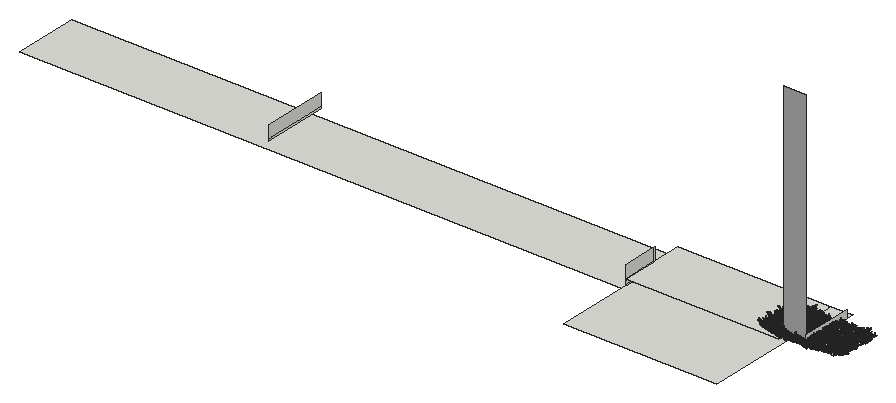
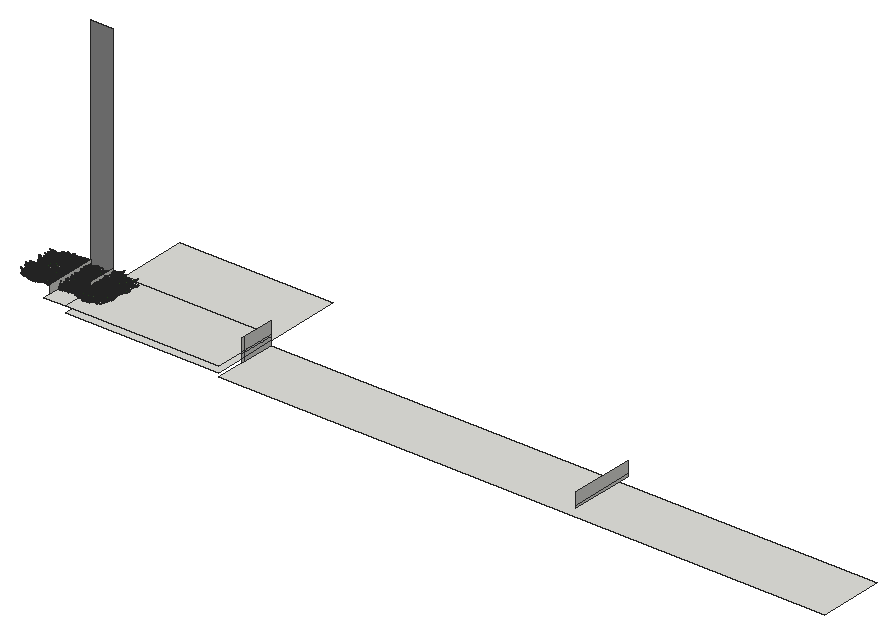
# SketchUp Ruby script. Lengths in inches.
U = 1.inch
M = Sketchup.active_model
def pt(a) = Geom::Point3d.new(a.map { |v| v * U })
def face(e, loops, mat)
  f = e.add_face(loops[0].map { |a| pt(a) })
  loops[1..].each { |l| e.add_face(l.map { |a| pt(a) }).erase! }
  f.material = f.back_material = mat if mat
  f
end
# faces: each face lists its corners as indices into pts; further lists are holes
def faces(e, pts, list, mat = nil) = list.each { |f| face(e, (f[0].is_a?(Array) ? f : [f]).map { |l| l.map { |i| pts[i] } }, mat) }
# xy, xz, yz: faces in a plane at the given z, y or x. An outline is a flat list of corners, or four numbers for a rectangle; further outlines are holes
def ring(l) = l.size == 4 ? [[l[0], l[1]], [l[2], l[1]], [l[2], l[3]], [l[0], l[3]]] : l.each_slice(2).to_a
def flat(e, list, mat, &to3) = list.each { |f| face(e, (f[0].is_a?(Array) ? f : [f]).map { |l| ring(l).map { |u, v| to3.(u, v) } }, mat) }
def xy(e, z, list, mat = nil) = flat(e, list, mat) { |x, y| [x, y, z] }
def xz(e, y, list, mat = nil) = flat(e, list, mat) { |x, z| [x, y, z] }
def yz(e, x, list, mat = nil) = flat(e, list, mat) { |y, z| [x, y, z] }
def lines(e, pts, list) = list.each { |a, b| e.add_line(pt(pts[a]), pt(pts[b])) }
# prism: a flat outline (further loops are holes) pulled along v
def prism(e, loops, v, mat = nil)
  f = face(e, loops, mat); d = Geom::Vector3d.new(v.map { |x| x * U })
  f.pushpull(f.normal.samedirection?(d) ? d.length : -d.length)
end
def box(e, o, s, mat = nil) = prism(e, [[o, [o[0] + s[0], o[1], o[2]], [o[0] + s[0], o[1] + s[1], o[2]], [o[0], o[1] + s[1], o[2]]]], [0, 0, s[2]], mat)
def at(x, y, z, deg = 0) = Geom::Transformation.translation(pt([x, y, z])) * Geom::Transformation.rotation(ORIGIN, Z_AXIS, deg.degrees)
def axes(o, x, y, z) = Geom::Transformation.new([*x, 0, *y, 0, *z, 0, *pt(o).to_a, 1])
def part(name) = M.definitions.add(name)
# library, detail: a bought-in or finely detailed component or shape, given as its bounding box
def library(name, o, s) = part(name).tap { |d| box(d.entities, o, s) }
def detail(e, o, s) = box(e.add_group.entities, o, s)
def put(e, d, t, mat = nil) = e.add_instance(d, t).tap { |i| i.material = mat if mat }
def group(e, t, mat = nil) = e.add_group.tap { |g| g.transformation = t; g.material = mat if mat }.entities
root = M.entities
M.materials.add("Material82").color = [68, 110, 58]
M.materials.add("Material83").color = [48, 90, 38]
M.materials.add("Material84").color = [68, 110, 48]
M.materials.add("Material85").color = [48, 90, 48]
M.materials.add("Material86").color = [58, 110, 58]
M.materials.add("Material87").color = [58, 90, 38]
M.materials.add("Material88").color = [68, 100, 58]
M.materials.add("Material89").color = [48, 100, 38]
M.materials.add("[Color M03]1").color = [170, 170, 170]
c1 = part("grass00")
p = [[-0.6875,0.15,0],[-0.56,0.08,5.52],[-0.04,0.03,2.76],[0.48,-0.02,0],[0.35,-0.02,5.52],[-0.1,-0.14,5.52],
  [-0.12,0.65,8.37],[-0.42,0.65,8.37]]
faces(c1.entities,p,[[0,1,2,3],[3,2,4],[1,5,2],[5,4,2],[1,6,5],[4,5,6],[7,6,1]])
c2 = part("Group16\#1")
put(c2.entities,c1,axes([1.44,-0.61,-0.01],[0.05352,0.12609,0],[-0.10704,0.04543,0.07239],[0.06664,-0.02828,0.11628]),"Material85")
put(c2.entities,c1,axes([0.76,-0.15,-0.01],[0.04676,0.24062,0],[-0.23162,0.04501,0.06642],[0.0652,-0.01267,0.23595]),"Material82")
put(c2.entities,c1,axes([0.79,0.01,-0.01],[-0.00606,0.34651,0],[-0.34381,-0.00602,0.0432],[0.04319,0.00076,0.34386]))
put(c2.entities,c1,axes([1,0.23,-0.01],[-0.07192,0.31144,0],[-0.28722,-0.06632,0.1236],[0.12043,0.02781,0.29478]),"Material84")
put(c2.entities,c1,axes([1.66,0.77,-0.01],[-0.13828,0.29651,0],[-0.21551,-0.1005,0.22471],[0.20365,0.09498,0.23779]),"Material89")
put(c2.entities,c1,axes([0.6875,0.52,-0.01],[-0.18126,0.24051,0],[-0.22746,-0.17142,0.09788],[0.07817,0.05891,0.28481]),"Material84")
put(c2.entities,c1,axes([0.68,0.78,-0.01],[-0.215,0.18688,0],[-0.12385,-0.14248,0.21334],[0.13995,0.16101,0.18878]),"Material82")
put(c2.entities,c1,axes([0.56,1,-0.01],[-0.13756,0.07624,0],[-0.06159,-0.11112,0.0927],[0.04494,0.08108,0.12705]),"Material84")
put(c2.entities,c1,axes([0.2,0.64,-0.01],[-0.23729,0.07254,0],[-0.05711,-0.18681,0.153],[0.04473,0.14632,0.19535]),"Material89")
put(c2.entities,c1,axes([0.0625,0.72,-0.01],[-0.28874,0.02525,0],[-0.02179,-0.24916,0.14647],[0.01276,0.14591,0.25012]),"Material82")
put(c2.entities,c1,axes([-0.08,0.62,-0.01],[-0.34089,-0.04187,0],[0.03255,-0.26504,0.216],[-0.02633,0.21439,0.26703]),"Material89")
put(c2.entities,c1,axes([-0.34,0.98,-0.01],[-0.14314,-0.0493,0],[0.04397,-0.12769,0.06843],[-0.02228,0.0647,0.13505]),"Material89")
put(c2.entities,c1,axes([-0.87,1.45,-0.01],[-0.23488,-0.14114,0],[0.13761,-0.22901,0.06087],[-0.03135,0.05217,0.26717]))
put(c2.entities,c1,axes([-0.72,0.77,-0.01],[-0.14208,-0.13251,0],[0.07209,-0.0773,0.16301],[-0.11118,0.11922,0.1057]),"Material89")
put(c2.entities,c1,axes([-0.62,0.43,-0.01],[-0.14845,-0.21203,0],[0.18654,-0.13061,0.12304],[-0.10079,0.07057,0.22772]),"Material82")
put(c2.entities,c1,axes([-0.68,0.29,-0.01],[-0.13639,-0.32136,0],[0.31723,-0.13464,0.05579],[-0.05136,0.0218,0.34462]),"Material83")
put(c2.entities,c1,axes([-0.64,0.125,-0.01],[-0.0458,-0.23569,0],[0.22124,-0.043,0.08276],[-0.08124,0.01579,0.22538]),"Material86")
put(c2.entities,c1,axes([-1.6,-0.03,-0.01],[0.00576,-0.32897,0],[0.27526,0.00482,0.18018],[-0.18015,-0.00315,0.2753]),"Material84")
put(c2.entities,c1,axes([-1.36,-0.31,-0.01],[0.05718,-0.24765,0],[0.18172,0.04196,0.17267],[-0.16825,-0.03885,0.1865]),"Material89")
put(c2.entities,c1,axes([-1.54,-0.72,-0.01],[0.06537,-0.14017,0],[0.13555,0.06321,0.03939],[-0.0357,-0.01665,0.14956]))
put(c2.entities,c1,axes([-1.19,-0.9,-0.01],[0.09597,-0.12735,0],[0.11214,0.08451,0.07557],[-0.06035,-0.04548,0.14042]),"Material88")
put(c2.entities,c1,axes([-0.47,-0.54,-0.01],[0.11588,-0.10072,0],[0.0618,0.0711,0.12124],[-0.07953,-0.0915,0.0942]))
put(c2.entities,c1,axes([-0.47,-0.84,-0.01],[0.11927,-0.0661,0],[0.06603,0.11913,0.00646],[-0.00313,-0.00565,0.13621]),"Material84")
put(c2.entities,c1,axes([-0.38,-1.24,-0.01],[0.28037,-0.08571,0],[0.0618,0.20215,0.20315],[-0.05939,-0.19428,0.21139]),"Material88")
put(c2.entities,c1,axes([-0.06,-0.66,-0.01],[0.22719,-0.01987,0],[0.01247,0.14255,0.17758],[-0.01547,-0.17691,0.1431]),"Material87")
put(c2.entities,c1,axes([0.11,-0.89,-0.01],[0.14882,0.01828,0],[-0.01058,0.08611,0.12229],[0.01491,-0.12138,0.08676]),"Material85")
put(c2.entities,c1,axes([0.25,-0.72,-0.01],[0.20481,0.07053,0],[-0.06206,0.18022,0.10291],[0.03351,-0.0973,0.1906]),"Material85")
put(c2.entities,c1,axes([0.85,-1.42,-0.01],[0.16481,0.09904,0],[-0.09472,0.15762,0.05616],[0.02893,-0.04814,0.18389]),"Material84")
put(c2.entities,c1,axes([1.01,-1.09,-0.01],[0.21858,0.20385,0],[-0.17495,0.1876,0.15339],[0.10462,-0.11218,0.25652]),"Material89")
put(c2.entities,c1,axes([1.01,-0.71,-0.01],[0.08733,0.12473,0],[-0.06445,0.04512,0.13037],[0.1068,-0.07477,0.07867]),"Material85")
c3 = part("Group15\#1")
put(c3.entities,c2,at(0,0,0))
c4 = part("3darcstudiotree_grass00\#1")
put(c4.entities,c3,at(0,0,0))
xy(root,-42.1875,[[1048.66,335.84,1534.73,387.84]])
xy(root,-39.125,[[1534.73,273.41,1657.41,387.84]])
xy(root,-34.17,[[1534.73,335.84,1657.41,387.84],[1657.41,341.03,1674.99,387.84]])
xz(root,341.03,[[1657.41,-34.17,1674.99,144.9375]],"[Color M03]1")
yz(root,1248.34,[[335.84,-35.625,387.84,-34.17],[335.84,-34.17,387.84,-24.25]])
yz(root,1534.73,[[335.84,-42.1875,362.97,-39.125],[362.97,-42.1875,364.46,-39.125],[335.84,-39.125,362.97,-35.625],[362.97,-39.125,364.46,-35.625],[335.84,-35.625,362.97,-34.17],
  [362.97,-35.625,364.46,-34.17],[335.84,-34.17,362.97,-24.25],[362.97,-34.17,364.46,-24.25]])
yz(root,1657.41,[[341.03,-34.17,362.97,-27.66]])
yz(root,1674.99,[[341.03,-34.17,381.72,-27.66]])
put(root,c4,axes([1645.09,350.95,-34.17],[-3.06097,-0.5879,0],[1.66705,-1.34995,-0.03924],[0.1162,-0.0941,1.93013]))
put(root,c4,axes([1646.65,355.5625,-34.17],[-4.03652,-0.16228,0],[0.44348,-1.71564,-0.03002],[0.01485,-0.05745,1.59842]))
put(root,c4,axes([1646.35,360.35,-34.17],[2.89762,-1.1399,0],[2.43274,0.96179,-0.0036],[0.01556,0.00615,1.5794]))
put(root,c4,axes([1646.26,342.71,-34.17],[3.9501,-0.3019,0],[0.82816,1.68526,-0.01483],[0.01308,0.02661,1.51152]))
put(root,c4,axes([1645.96,364.46,-34.17],[3.35543,0.83331,0],[-2.02345,1.2672,-0.03908],[-0.13338,0.08353,1.82303]))
put(root,c4,axes([1646.7,348.62,-34.17],[2.855,1.42821,0],[-2.79418,0.86872,-0.04305],[-0.19263,0.05989,1.51958]))
put(root,c4,axes([1648.4,371.03,-34.17],[4.14496,0.31804,0],[-0.83759,1.6978,-0.03864],[-0.04159,0.0843,1.85268]))
put(root,c4,axes([1648.57,342.22,-34.17],[3.14768,1.20624,0],[-3.13864,1.27383,-0.06236],[-0.23969,0.09728,1.86199]))
put(root,c4,axes([1649.89,367.78,-34.17],[1.22629,-1.22817,0],[3.78204,0.58732,-0.0431],[0.18193,0.02825,1.38217]))
put(root,c4,axes([1649.94,354.84,-34.17],[2.09831,-1.02697,0],[3.53268,1.1226,-0.04335],[0.15343,0.04876,1.54559]))
put(root,c4,axes([1649.82,351.3,-34.17],[-2.72452,1.24598,0],[-3.55259,-1.2082,-0.04683],[-0.18808,-0.06396,1.86493]))
put(root,c4,axes([1649.3,357.3125,-34.17],[3.77194,0.53127,0],[-1.56854,1.73204,-0.02984],[-0.04464,0.0493,1.55474]))
put(root,c4,axes([1650.93,353.18,-34.17],[0.71144,-1.32945,0],[4.31841,0.35942,-0.04294],[0.17046,0.01419,1.34209]))
put(root,c4,axes([1651.22,360.26,-34.17],[1.7149,-1.22637,0],[3.67075,0.79833,-0.00061],[0.00329,0.00072,1.94394]))
put(root,c4,axes([1651.55,362.27,-34.17],[1.13517,-1.33714,0],[4.08386,0.53922,-0.04023],[0.16123,0.02129,1.36415]))
put(root,c4,axes([1650.625,366.27,-34.17],[-1.96155,1.42232,0],[-3.86474,-0.82896,-0.01158],[-0.04562,-0.00979,1.47884]))
put(root,c4,axes([1652.02,372.46,-34.17],[-0.47401,-1.83018,0],[3.81106,-0.15352,-0.01024],[0.06486,-0.00261,1.82793]))
put(root,c4,axes([1651.45,363.91,-34.17],[-2.22727,1.60419,0],[-4.12877,-0.89155,-0.00813],[-0.02667,-0.00576,1.31962]))
put(root,c4,axes([1651.8,348.36,-34.17],[-2.60888,1.40075,0],[-3.4553,-1.0009,-0.02364],[-0.11495,-0.0333,1.93862]))
put(root,c4,axes([1652.17,347.26,-34.17],[3.43972,-1.19732,0],[3.07284,1.37298,-0.00351],[0.01073,0.00479,1.60808]))
put(root,c4,axes([1652.2,344.94,-34.17],[2.57433,-1.10368,0],[3.03991,1.10279,-0.05921],[0.27011,0.09799,1.91907]))
put(root,c4,axes([1654.11,364.41,-34.17],[-1.00872,-1.50256,0],[3.76018,-0.39261,-0.00114],[0.00668,-0.0007,1.77079]))
put(root,c4,axes([1654.41,351.03,-34.17],[-4.39065,-0.68044,0],[1.48247,-1.48779,-0.03326],[0.06181,-0.06203,1.54402]))
put(root,c4,axes([1654.4,365.79,-34.17],[-4.44259,0.07323,0],[-0.15396,-1.45277,-0.02048],[-0.00618,-0.05831,1.99696]))
put(root,c4,axes([1653.9,361.58,-34.17],[-2.76199,0.84111,0],[-2.40625,-1.22891,-0.02049],[-0.06035,-0.03082,1.42185]))
put(root,c4,axes([1654.5,344.48,-34.17],[4.22079,-0.16227,0],[0.44484,1.79962,-0.00515],[0.00263,0.01065,1.80879]))
put(root,c4,axes([1656.62,341.46,-34.17],[-4.16244,-0.15093,0],[0.36502,-1.56574,-0.01686],[0.00714,-0.03063,1.38194]))
put(root,c4,axes([1655.3,358.125,-34.17],[-0.6643,1.32662,0],[-4.47997,-0.3489,-0.01512],[-0.08059,-0.00628,1.85999]))
put(root,c4,axes([1656.86,349.27,-34.17],[0.943,-1.41783,0],[3.80413,0.39351,-0.01105],[0.05525,0.00572,1.52421]))
put(root,c4,axes([1655.42,340.13,-34.17],[0.93193,1.68006,0],[-3.63506,0.3136,-0.00261],[-0.01526,0.00132,1.6704]))
put(root,c4,axes([1657.5,355.56,-34.17],[-3.93808,-0.75827,0],[2.05575,-1.66052,-0.06565],[0.13947,-0.11266,1.70067]))
put(root,c4,axes([1655.9,359.26,-34.17],[-0.07538,1.68656,0],[-4.43832,-0.03085,-0.00958],[-0.0427,-0.0003,1.48335]))
put(root,c4,axes([1656.73,347.11,-34.17],[0.31598,1.50106,0],[-3.48689,0.11416,-0.00998],[-0.05116,0.00168,1.34846]))
put(root,c4,axes([1657.55,371.18,-34.17],[3.02082,-1.15648,0],[2.42176,0.98385,-0.02978],[0.11407,0.04634,1.43312]))
put(root,c4,axes([1657,367.64,-34.17],[3.58704,0.55594,0],[-1.39662,1.40151,-0.02634],[-0.05335,0.05353,1.58474]))
put(root,c4,axes([1657.63,352.21,-34.17],[3.13564,-0.95157,0],[2.13614,1.09478,-0.03629],[0.11919,0.06109,1.41389]))
put(root,c4,axes([1659.5,369.84,-34.17],[-3.8239,-0.32025,0],[0.87863,-1.63166,-0.02543],[0.02678,-0.04974,1.60712]))
put(root,c4,axes([1660.31,364.32,-34.17],[-1.37854,-1.47975,0],[3.2131,-0.46555,-0.02344],[0.115,-0.01666,1.34096]))
put(root,c4,axes([1660.08,346.58,-34.17],[-3.58928,0.33039,0],[-0.75882,-1.28211,-0.0198],[-0.02657,-0.04489,1.47686]))
put(root,c4,axes([1659.91,366.04,-34.17],[1.03001,-1.55898,0],[3.46185,0.35573,-0.04641],[0.24674,0.02535,1.47323]))
put(root,c4,axes([1660.66,361.51,-34.17],[0.07037,-1.71405,0],[4.70144,0.03002,-0.02796],[0.12644,0.00081,1.59394]))
put(root,c4,axes([1660.77,358.96,-34.17],[-4.25189,0.62806,0],[-1.17044,-1.23238,-0.01358],[-0.02814,-0.02963,1.47772]))
put(root,c4,axes([1661.13,357.41,-34.17],[-4.15804,-0.01553,0],[0.04454,-1.85443,-0.04475],[0.00172,-0.0718,1.43393]))
put(root,c4,axes([1661.33,355.67,-34.17],[-3.68076,-0.30441,0],[0.87866,-1.65237,-0.00999],[0.00884,-0.01661,1.38276]))
put(root,c4,axes([1660.97,369.11,-34.17],[-2.36198,1.34531,0],[-2.91809,-0.79683,-0.03104],[-0.17128,-0.04677,1.78553]))
put(root,c4,axes([1661.4375,344.33,-34.17],[2.97125,-1.188,0],[2.63587,1.02532,-0.00165],[0.00768,0.00299,1.81884]))
put(root,c4,axes([1662.48,339.87,-34.17],[-1.66901,-1.67644,0],[3.86369,-0.59826,-0.05278],[0.29329,-0.04541,1.85719]))
put(root,c4,axes([1662.59,341.39,-34.17],[-4.35861,-0.14504,0],[0.36663,-1.71363,-0.02802],[0.01298,-0.06068,1.8014]))
put(root,c4,axes([1661.29,352.64,-34.17],[3.6615,0.00284,0],[-0.00662,1.32579,-0.0306],[-0.00046,0.09111,1.9022]))
put(root,c4,axes([1662.7,351.26,-34.17],[-3.40532,-0.07402,0],[0.22612,-1.61806,-0.00601],[0.00193,-0.01379,1.79325]))
put(root,c4,axes([1661.69,349.14,-34.17],[3.15923,1.14894,0],[-3.00225,1.28393,-0.03053],[-0.12215,0.05224,1.95907]))
put(root,c4,axes([1664.73,341.86,-34.17],[3.82244,-0.70635,0],[1.81239,1.52539,-0.00986],[0.01787,0.01504,1.36783]))
put(root,c4,axes([1665.69,359.25,-34.17],[-3.50881,1.16011,0],[-2.69176,-1.26622,-0.04843],[-0.14054,-0.06611,1.41858]))
put(root,c4,axes([1665.08,353.67,-34.17],[3.5983,-0.42057,0],[0.96573,1.28508,-0.03127],[0.05191,0.06908,1.48816]))
put(root,c4,axes([1665.09,351.11,-34.17],[-1.39865,1.66077,0],[-3.78259,-0.49545,-0.00679],[-0.0282,-0.00369,1.30662]))
put(root,c4,axes([1665.89,364.09,-34.17],[2.65926,-1.384,0],[3.07673,0.91944,-0.04967],[0.23773,0.07104,1.73743]))
put(root,c4,axes([1665.27,346.05,-34.17],[3.23293,0.85538,0],[-2.19162,1.28829,-0.0468],[-0.14196,0.08345,1.60535]))
put(root,c4,axes([1666.39,370.58,-34.17],[-1.23102,1.43236,0],[-4.00109,-0.53481,-0.05878],[-0.24424,-0.03265,1.38915]))
put(root,c4,axes([1667.66,368.61,-34.17],[-3.85586,-0.61181,0],[1.38378,-1.3564,-0.02256],[0.04705,-0.04612,1.55256]))
put(root,c4,axes([1666.18,365.61,-34.17],[4.58666,-0.29954,0],[0.76961,1.83286,-0.06031],[0.05541,0.13196,1.9859]))
put(root,c4,axes([1665.89,356.65,-34.17],[2.59618,1.43862,0],[-2.87173,0.80602,-0.01154],[-0.04691,0.01317,1.31865]))
put(root,c4,axes([1667.42,344.33,-34.17],[0.50435,-1.60129,0],[3.80498,0.18639,-0.05019],[0.26525,0.01299,1.53052]))
put(root,c4,axes([1666.72,362.3,-34.17],[3.24935,0.42764,0],[-1.43334,1.69386,-0.04175],[-0.05922,0.06999,1.52086]))
put(root,c4,axes([1667.09,348.15,-34.17],[4.09406,-0.23131,0],[0.47213,1.29969,-0.032],[0.03631,0.09996,1.99674]))
put(root,c4,axes([1667.52,340.25,-34.17],[1.78223,1.25772,0],[-3.10123,0.68348,-0.02391],[-0.11693,0.02577,1.49173]))
put(root,c4,axes([1667.53,355.03,-34.17],[0.65139,1.7147,0],[-4.45072,0.26296,-0.01905],[-0.08769,0.00518,1.57029]))
put(root,c4,axes([1670.81,370.89,-34.17],[-3.04991,-1.12114,0],[2.90905,-1.23081,-0.00052],[0.00199,-0.00084,1.79691]))
put(root,c4,axes([1672.46,368.53,-34.17],[0.23876,-1.55199,0],[4.36064,0.10434,-0.04584],[0.18368,0.0044,1.3146]))
put(root,c4,axes([1672.72,351.125,-34.17],[-0.00481,-1.55543,0],[4.64446,-0.00224,-0.02113],[0.08601,-0.00004,1.41674]))
put(root,c4,axes([1671.39,344.05,-34.17],[3.47227,-0.30693,0],[0.74979,1.31925,-0.01015],[0.01336,0.0235,1.54623]))
put(root,c4,axes([1671.36,346.05,-34.17],[-1.26342,1.38148,0],[-3.54227,-0.50384,-0.00809],[-0.04856,-0.00691,1.80065]))
put(root,c4,axes([1672,352.72,-34.17],[2.94151,-0.90679,0],[2.69176,1.35804,-0.00613],[0.02014,0.01016,1.74641]))
put(root,c4,axes([1671.27,365.35,-34.17],[0.11831,1.37685,0],[-3.50344,0.04682,-0.00216],[-0.01444,0.00019,1.758]))
put(root,c4,axes([1672.92,356.01,-34.17],[-0.73982,-1.44093,0],[3.74487,-0.29904,-0.04711],[0.2431,-0.01941,1.50792]))
put(root,c4,axes([1672.41,361.35,-34.17],[2.48182,-1.04217,0],[2.75852,1.02169,-0.02466],[0.10108,0.03744,1.59511]))
put(root,c4,axes([1672.25,348.7,-34.17],[-2.81085,1.01922,0],[-2.91901,-1.25203,-0.0061],[-0.02341,-0.01004,1.83281]))
put(root,c4,axes([1672.18,341.63,-34.17],[-0.96185,1.4826,0],[-3.70839,-0.37418,-0.04208],[-0.21883,-0.02208,1.54007]))
put(root,c4,axes([1673.65,359.52,-34.17],[-0.3225,-1.34219,0],[4.58247,-0.17125,-0.03587],[0.16603,-0.0062,1.60406]))
put(root,c4,axes([1672.38,340.65,-34.17],[3.91343,0.66663,0],[-1.38696,1.26634,-0.02193],[-0.04877,0.04453,1.47013]))
put(root,c4,axes([1673.2,363.84,-34.17],[3.82293,-1.07301,0],[2.00012,1.10831,-0.02041],[0.08948,0.04958,1.95445]))
put(root,c4,axes([1673.06,357.49,-34.17],[3.70183,0.03147,0],[-0.07805,1.42775,-0.0399],[-0.00598,0.10931,1.8861]))
put(root,c4,axes([1676.74,354.69,-34.17],[-0.79677,-1.6402,0],[3.36468,-0.25421,-0.01579],[0.08769,-0.00662,1.45182]))
put(root,c4,axes([1677.25,350.28,-34.17],[-4.49567,-0.3985,0],[0.83225,-1.46029,-0.03373],[0.03467,-0.06083,1.33323]))
put(root,c4,axes([1677.17,352.49,-34.17],[-4.6805,0.28538,0],[-0.54089,-1.37973,-0.03554],[-0.03758,-0.09587,1.83631]))
put(root,c4,axes([1675.9,358.97,-34.17],[-0.10316,1.55622,0],[-4.09748,-0.04224,-0.03889],[-0.19104,-0.00197,1.50954]))
put(root,c4,axes([1676.71,356.86,-34.17],[-3.29804,1.27107,0],[-2.52678,-1.01968,-0.01484],[-0.07094,-0.02863,1.85373]))
put(root,c4,axes([1676.85,363.52,-34.17],[2.48968,-1.1461,0],[2.93182,0.99053,-0.00664],[0.0258,0.00872,1.48048]))
put(root,c4,axes([1678.29,368.03,-34.17],[-1.20508,-1.27416,0],[3.97727,-0.58504,-0.0406],[0.22085,-0.03249,1.84742]))
put(root,c4,axes([1677.4375,346.98,-34.17],[-0.56456,1.41966,0],[-3.50259,-0.21664,-0.01794],[-0.10644,-0.00658,1.59592]))
put(root,c4,axes([1677.42,366.93,-34.17],[1.96349,1.64722,0],[-3.56633,0.66117,-0.03464],[-0.18907,0.03505,1.78143]))
put(root,c4,axes([1679.67,340.02,-34.17],[-2.26232,-1.46372,0],[3.35674,-0.80691,-0.05337],[0.23381,-0.0562,1.5119]))
put(root,c4,axes([1679.22,361.32,-34.17],[2.10633,-1.56652,0],[4.07545,0.85227,-0.05067],[0.19625,0.04104,1.51576]))
put(root,c4,axes([1679.13,341.8,-34.17],[2.08347,-1.59715,0],[3.15506,0.64012,-0.03693],[0.21917,0.04447,1.77491]))
put(root,c4,axes([1678.18,348.7,-34.17],[0.79004,1.45858,0],[-4.26548,0.35933,-0.00171],[-0.00893,0.00075,1.74655]))
put(root,c4,axes([1679.89,371.06,-34.17],[1.69514,-1.26112,0],[3.85825,0.80658,-0.01977],[0.09529,0.01992,1.78562]))
put(root,c4,axes([1678.75,343.68,-34.17],[3.33408,0.32893,0],[-1.10916,1.74856,-0.00744],[-0.00738,0.01164,1.4009]))
put(root,c4,axes([1682.46,348.7,-34.17],[-4.09965,-0.15274,0],[0.36855,-1.53851,-0.03137],[0.01329,-0.05547,1.3228]))
put(root,c4,axes([1681.91,366.12,-34.17],[-3.21191,1.28173,0],[-2.59769,-1.01243,-0.03007],[-0.15402,-0.06003,1.97134]))
put(root,c4,axes([1682.91,356.73,-34.17],[-1.51918,-1.57572,0],[4.39344,-0.65879,-0.02869],[0.10716,-0.01607,1.40786]))
put(root,c4,axes([1683.29,341.9,-34.17],[-4.22007,0.35003,0],[-0.86715,-1.62599,-0.01674],[-0.0198,-0.03713,1.81501]))
put(root,c4,axes([1682.66,361.08,-34.17],[-1.69964,1.49974,0],[-3.25198,-0.57319,-0.0353],[-0.21623,-0.03811,1.79152]))
put(root,c4,axes([1682.62,360.03,-34.17],[-1.65501,1.23077,0],[-2.99443,-0.62625,-0.02105],[-0.13776,-0.02881,1.88169]))
put(root,c4,axes([1681.95,346.7,-34.17],[3.27704,0.72692,0],[-1.98468,1.39155,-0.00275],[-0.00611,0.00428,1.37565]))
put(root,c4,axes([1683.89,350.27,-34.17],[-2.87872,-0.88154,0],[2.80816,-1.42624,-0.06125],[0.14894,-0.07565,1.36064]))
put(root,c4,axes([1683.45,355.28,-34.17],[0.11814,-1.8536,0],[3.92163,0.03887,-0.05528],[0.30038,0.00298,1.59813]))
put(root,c4,axes([1684.81,364.48,-34.17],[-1.1098,-1.31734,0],[3.29231,-0.43138,-0.00285],[0.02011,-0.00264,1.93438]))
put(root,c4,axes([1684.78,353.16,-34.17],[-2.16844,-1.41891,0],[2.90956,-0.69156,-0.03107],[0.17396,-0.04135,1.66455]))
put(root,c4,axes([1685,369.03,-34.17],[-3.85239,-0.20163,0],[0.58764,-1.74619,-0.01228],[0.0079,-0.02349,1.63767]))
put(root,c4,axes([1685.06,370.22,-34.17],[-1.66799,1.12199,0],[-3.57556,-0.82672,-0.01566],[-0.07039,-0.01628,1.61828]))
put(root,c4,axes([1685.16,344.16,-34.17],[3.70469,-0.86578,0],[1.68851,1.12372,-0.02001],[0.07058,0.04697,1.71774]))
put(root,c4,axes([1689.49,369.12,-34.17],[-4.16983,-0.88311,0],[1.85574,-1.3628,-0.02099],[0.05036,-0.03698,1.49075]))
put(root,c4,axes([1688.71,351.28,-34.17],[2.24844,-1.02464,0],[3.26531,1.11441,-0.03846],[0.14191,0.04843,1.57923]))
put(root,c4,axes([1689.47,370.01,-34.17],[-1.93961,-1.1589,0],[2.81158,-0.73187,-0.03406],[0.19491,-0.05074,1.73123]))
put(root,c4,axes([1689.82,348.88,-34.17],[-2.17228,-1.46024,0],[3.41853,-0.79094,-0.03431],[0.15337,-0.03548,1.53951]))
put(root,c4,axes([1689.15,361.59,-34.17],[2.63669,-1.45672,0],[3.66232,1.03098,-0.04124],[0.15536,0.04373,1.56101]))
put(root,c4,axes([1688.65,360.14,-34.17],[3.40582,0.10745,0],[-0.34866,1.71886,-0.00093],[-0.00031,0.0015,1.35201]))
put(root,c4,axes([1688.37,346.68,-34.17],[4.00271,0.72936,0],[-1.54017,1.31459,-0.00765],[-0.0159,0.01357,1.36419]))
put(root,c4,axes([1690.2,365.68,-34.17],[0.50947,-1.51274,0],[4.49668,0.23554,-0.03191],[0.15996,0.00838,1.71939]))
put(root,c4,axes([1690.45,342.24,-34.17],[-4.17152,-0.5223,0],[1.23744,-1.53711,-0.0262],[0.03523,-0.04376,1.36239]))
put(root,c4,axes([1690.44,354.41,-34.17],[-3.49855,-0.51529,0],[1.58914,-1.67809,-0.03885],[0.07118,-0.07517,1.78292]))
put(root,c4,axes([1688.72,363.2,-34.17],[-0.28743,1.31478,0],[-4.42266,-0.15037,-0.00545],[-0.03167,-0.00108,1.93955]))
put(root,c4,axes([1690.87,356.97,-34.17],[-3.86459,-0.0799,0],[0.17825,-1.34085,-0.00586],[0.00206,-0.0155,1.71352]))
put(root,c4,axes([1689.44,353.04,-34.17],[0.76665,1.71699,0],[-3.34963,0.23261,-0.02162],[-0.1104,0.00767,1.32159]))
put(root,c4,axes([1690.7,344.93,-34.17],[3.46997,0.08994,0],[-0.27266,1.63611,-0.01423],[-0.00549,0.03292,1.83161]))
put(root,c4,axes([1692.95,342.63,-34.17],[-4.50934,-0.15911,0],[0.38591,-1.70103,-0.03473],[0.01636,-0.07211,1.7157]))
put(root,c4,axes([1693.63,356.79,-34.17],[-1.29023,-1.58759,0],[3.9469,-0.49888,-0.03893],[0.19606,-0.02478,1.64312]))
put(root,c4,axes([1693.89,359.51,-34.17],[-3.37238,-1.2695,0],[3.05865,-1.2637,-0.04863],[0.19789,-0.08176,1.95701]))
put(root,c4,axes([1693.63,368.54,-34.17],[0.71095,-1.43364,0],[4.62721,0.35689,-0.06032],[0.23627,0.01822,1.41053]))
put(root,c4,axes([1693.67,362.16,-34.17],[-3.5162,-0.01544,0],[0.03762,-1.33225,-0.02017],[0.00158,-0.05579,1.77597]))
put(root,c4,axes([1694.22,344.06,-34.17],[-2.35898,-1.49879,0],[3.37563,-0.82632,-0.02087],[0.09435,-0.0231,1.58468]))
put(root,c4,axes([1693.35,349.125,-34.17],[2.33704,1.50763,0],[-2.98263,0.71909,-0.02868],[-0.14145,0.0341,1.51486]))
put(root,c4,axes([1695.17,372.63,-34.17],[-0.8203,-1.58295,0],[4.36315,-0.35165,-0.03636],[0.17472,-0.01408,1.63697]))
put(root,c4,axes([1696.01,347.07,-34.17],[0.6786,-1.83556,0],[4.57598,0.26311,-0.00277],[0.01184,0.00068,1.49508]))
put(root,c4,axes([1694.52,369.6875,-34.17],[3.70622,-0.07941,0],[0.19617,1.42399,-0.02262],[0.0073,0.05302,1.6131]))
put(root,c4,axes([1694.65,350.86,-34.17],[2.20491,1.1875,0],[-2.92266,0.84401,-0.01948],[-0.09978,0.02881,1.72408]))
put(root,c4,axes([1696.22,364.14,-34.17],[-3.77729,0.83126,0],[-1.83032,-1.29355,-0.03544],[-0.09552,-0.06751,1.55733]))
put(root,c4,axes([1696.31,354.53,-34.17],[1.99944,-1.04992,0],[3.08282,0.91308,-0.00267],[0.01382,0.00409,1.87177]))
put(root,c4,axes([1696.47,366.61,-34.17],[-3.83744,0.33373,0],[-0.9251,-1.65441,-0.02531],[-0.02998,-0.05361,1.77094]))
put(root,c4,axes([1695.21,353.22,-34.17],[3.34663,1.11106,0],[-2.8307,1.32609,-0.01247],[-0.04541,0.02127,1.86292]))
